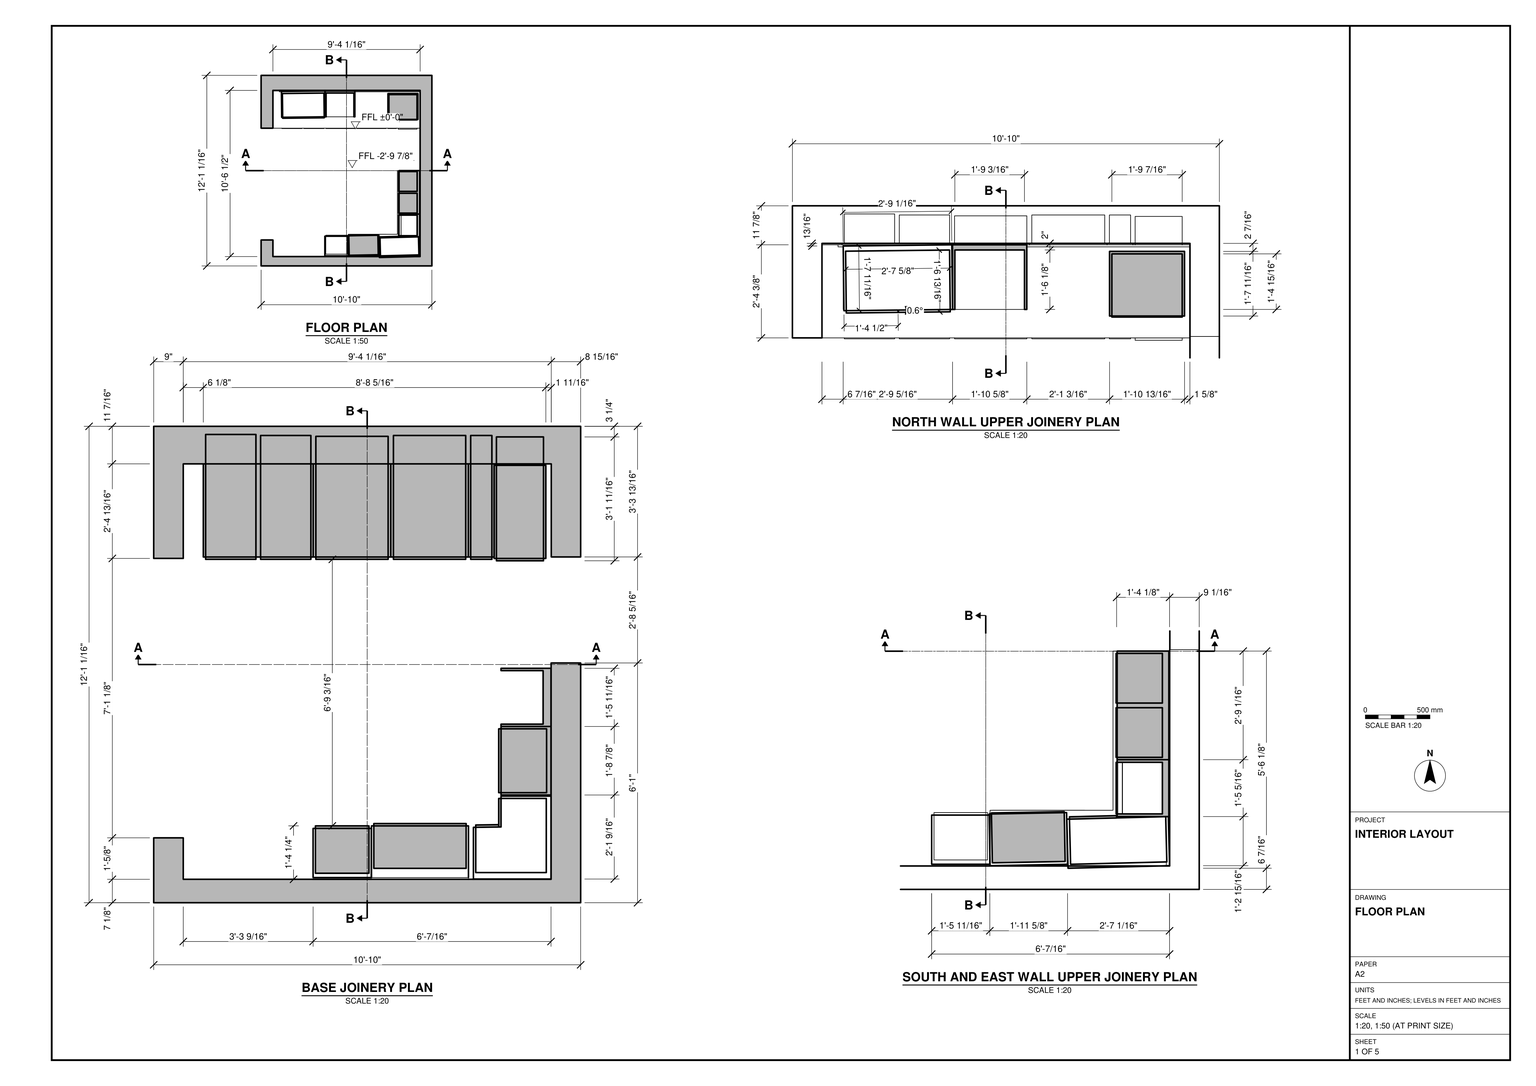
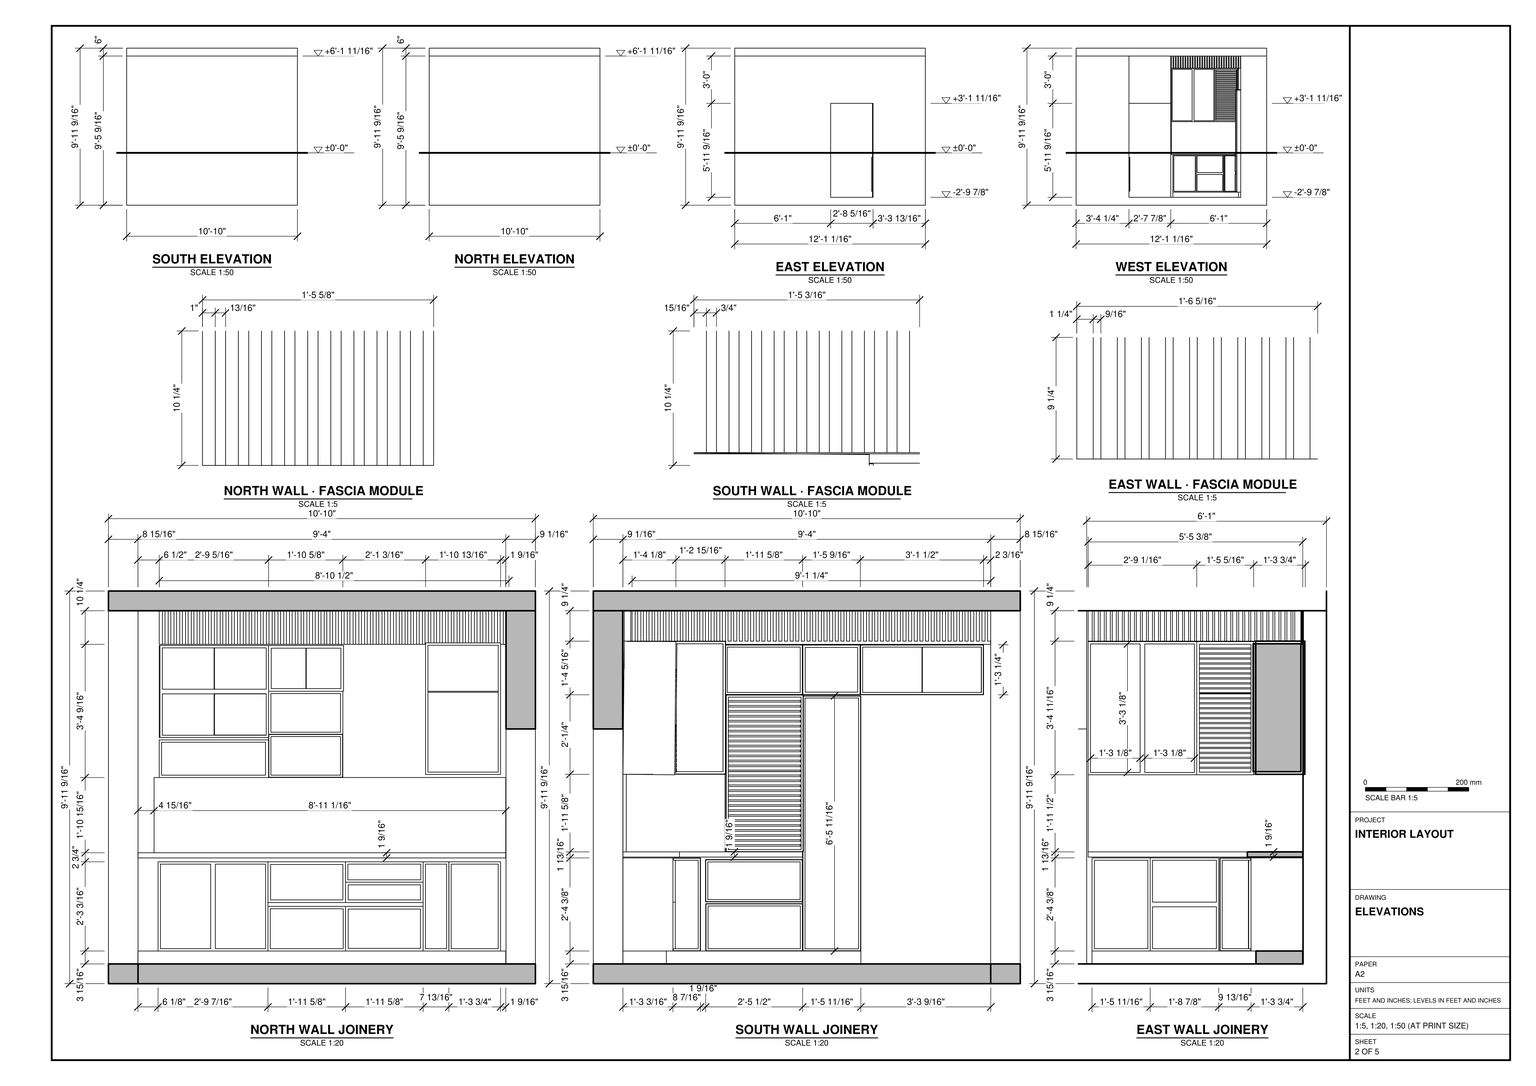
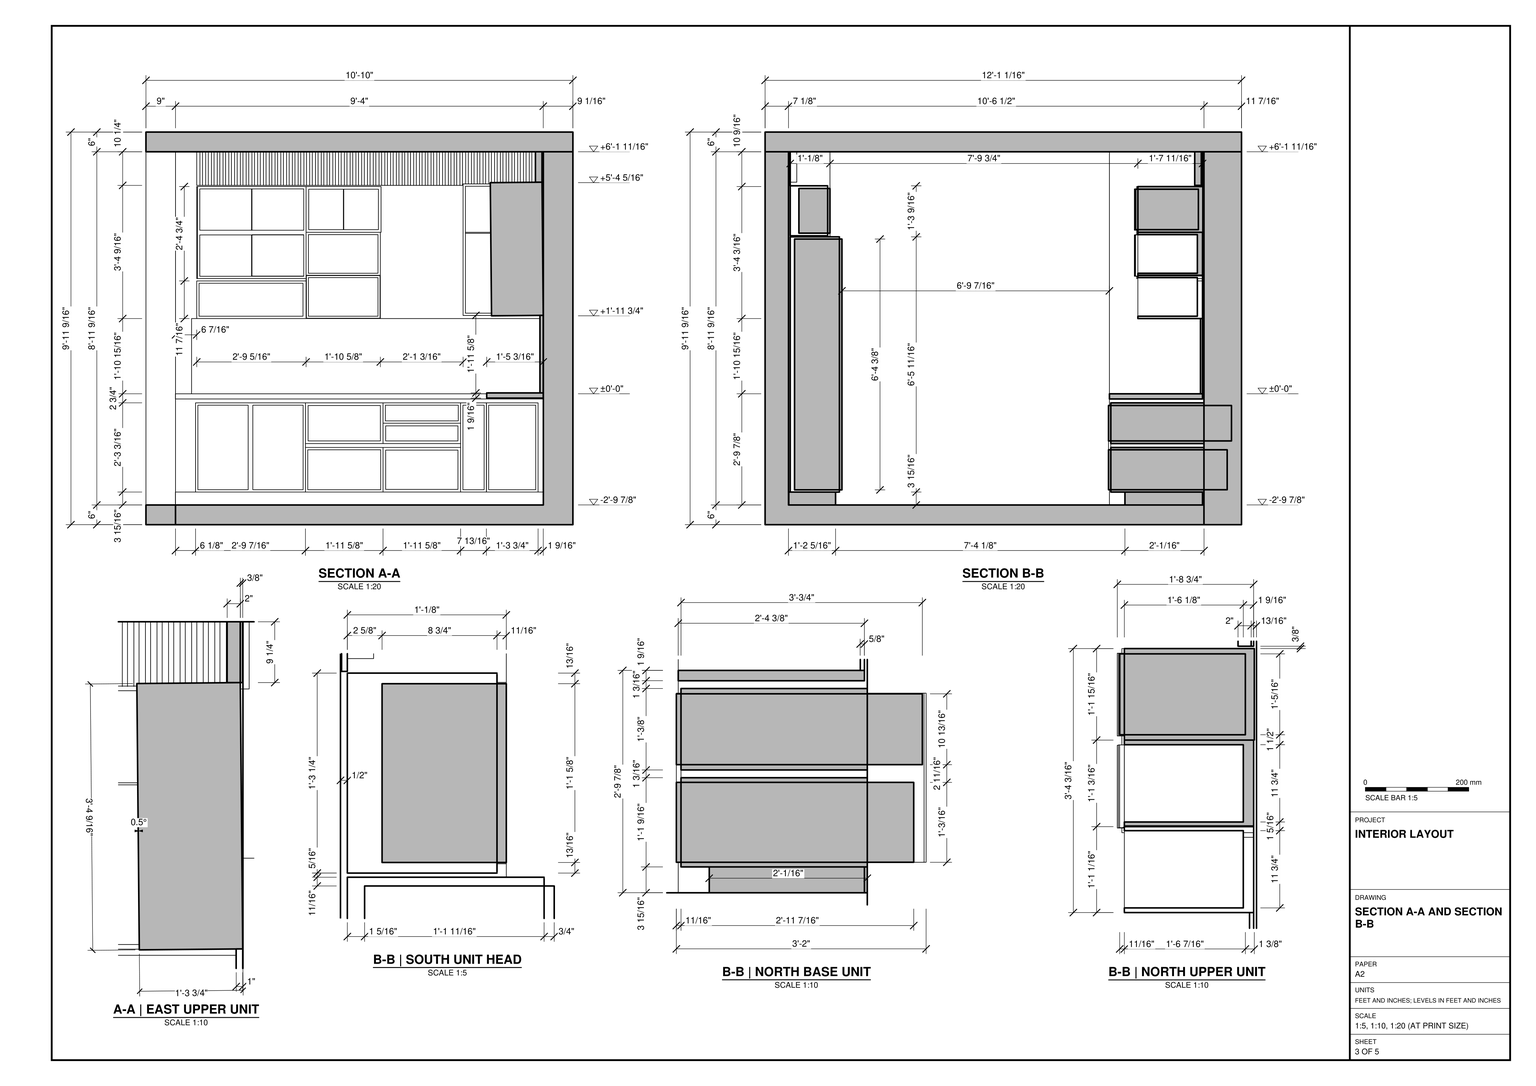
Build the room and its fitted cabinetry in SketchUp from task_files/diagram_01.pdf. Work in feet and inches. Set the outside dimensions to 10'-10" east to west, 12'-1 1/16" north to south and 9'-11 9/16" high. Use the single-storey datum ±0'-0" at the north worktop; the finished floor is at -2'-9 7/8" in the sections.

Model the floor slab, overhead slab and walls with their thicknesses as drawn. Leave the wide opening between the west wall returns and form the narrower opening in the east wall. Use the base and upper joinery plans separately: the cabinet footprints change with height. On the north wall, model the recessed plinth, base cabinets, drawer fronts and continuous worktop. Above it, build the divided upper cabinets and leave the gap before the right-hand unit. Fit the other cabinet run around the south-east corner, matching the tall unit, overhead cabinets and horizontally slatted fronts to the elevations. Distinguish those fronts from the vertically ribbed fascia above the cabinetry.

Keep the walls, slabs and each joinery piece in separate groups or components, and use components for repeated parts. Any decor or loose items shown may be represented by suitable library components. Save one SketchUp model as output_files/room_shell_and_three_wall_cabinet_fit_out.skp.

# SketchUp Ruby script. Lengths in inches.
U = 1.inch
M = Sketchup.active_model
def pt(a) = Geom::Point3d.new(a.map { |v| v * U })
def face(e, loops, mat)
  f = e.add_face(loops[0].map { |a| pt(a) })
  loops[1..].each { |l| e.add_face(l.map { |a| pt(a) }).erase! }
  f.material = f.back_material = mat if mat
  f
end
# faces: each face lists its corners as indices into pts; further lists are holes
def faces(e, pts, list, mat = nil) = list.each { |f| face(e, (f[0].is_a?(Array) ? f : [f]).map { |l| l.map { |i| pts[i] } }, mat) }
# xy, xz, yz: faces in a plane at the given z, y or x. An outline is a flat list of corners, or four numbers for a rectangle; further outlines are holes
def ring(l) = l.size == 4 ? [[l[0], l[1]], [l[2], l[1]], [l[2], l[3]], [l[0], l[3]]] : l.each_slice(2).to_a
def flat(e, list, mat, &to3) = list.each { |f| face(e, (f[0].is_a?(Array) ? f : [f]).map { |l| ring(l).map { |u, v| to3.(u, v) } }, mat) }
def xy(e, z, list, mat = nil) = flat(e, list, mat) { |x, y| [x, y, z] }
def xz(e, y, list, mat = nil) = flat(e, list, mat) { |x, z| [x, y, z] }
def yz(e, x, list, mat = nil) = flat(e, list, mat) { |y, z| [x, y, z] }
def lines(e, pts, list) = list.each { |a, b| e.add_line(pt(pts[a]), pt(pts[b])) }
# prism: a flat outline (further loops are holes) pulled along v
def prism(e, loops, v, mat = nil)
  f = face(e, loops, mat); d = Geom::Vector3d.new(v.map { |x| x * U })
  f.pushpull(f.normal.samedirection?(d) ? d.length : -d.length)
end
def box(e, o, s, mat = nil) = prism(e, [[o, [o[0] + s[0], o[1], o[2]], [o[0] + s[0], o[1] + s[1], o[2]], [o[0], o[1] + s[1], o[2]]]], [0, 0, s[2]], mat)
def at(x, y, z, deg = 0) = Geom::Transformation.translation(pt([x, y, z])) * Geom::Transformation.rotation(ORIGIN, Z_AXIS, deg.degrees)
def axes(o, x, y, z) = Geom::Transformation.new([*x, 0, *y, 0, *z, 0, *pt(o).to_a, 1])
def part(name) = M.definitions.add(name)
# library, detail: a bought-in or finely detailed component or shape, given as its bounding box
def library(name, o, s) = part(name).tap { |d| box(d.entities, o, s) }
def detail(e, o, s) = box(e.add_group.entities, o, s)
def put(e, d, t, mat = nil) = e.add_instance(d, t).tap { |i| i.material = mat if mat }
def group(e, t, mat = nil) = e.add_group.tap { |g| g.transformation = t; g.material = mat if mat }.entities
root = M.entities
M.materials.add("Teddy_Bracelet").color = [145, 141, 147]
M.materials.add("Teddy_DressDepth").color = [117, 194, 193]
M.materials.add("Teddy_Skin ").color = [196, 161, 133]
M.materials.add("[Color B03]").color = [201, 127, 109]
M.materials.add("[Color H06]").color = [158, 204, 204]
M.materials.add("[Color M00]").color = [255, 255, 255]
M.materials.add("[Color M04]").color = [142, 142, 142]
M.materials.add("[Metal Steel Textured]").color = [106, 110, 123]
M.materials.add("[Translucent Glass Sky Reflection]").color = [126, 138, 183]
M.materials["[Translucent Glass Sky Reflection]"].alpha = 0.52
M.materials.add("[Wood Veneer 01]").color = [120, 70, 37]
M.materials.add("[Wood Veneer 02]").color = [190, 128, 91]
c1 = part("Group\#46")
box(c1.entities,[0,-2,0],[0.97,2,10.24])
c2 = part("Group\#68")
box(c2.entities,[-2,0,0],[2,1.25,9.26])
c3 = part("Group\#58")
prism(c3.entities,[[[1.5,0,-0.15],[1.5,15.12,-0.15],[13.78,15.12,-0.04],[13.78,0,-0.04]]],[0,0,0.52])
c4 = part("Group\#62")
prism(c4.entities,[[[1.5,0,-0.34],[1.5,15.71,-0.34],[13.78,15.71,-0.23],[13.78,0,-0.23]]],[-0.01,0,0.71])
c5 = part("Group\#63")
g1 = group(c5.entities,at(0,0,0))
prism(g1,[[[0.01,15.71,0],[0.01,0,0],[-0.15,0,0],[-0.15,15.71,0]]],[-0.01,0,1.12])
c6 = part("Group\#75")
box(c6.entities,[0,0,0],[0.95,2,9.26])
c7 = part("Group\#84")
prism(c7.entities,[[[22.17,0.41,0],[0,0,0],[-0.01,0.31,0],[22.17,0.73,0]]],[0,0,1.04])
xy(root,4.08,[[8.97,109.58,15.07,133.2]])
p = [[66.32,7.22,82.11],[66.32,7.65,97.47],[89.91,7.65,97.47],[89.91,7.22,82.11]]
faces(root,p,[[0,1,2,3]])
g2 = group(root,at(8.97,95.84,0.14))
box(g2,[0,13.74,0],[112.01,23.62,3.9375])
g3 = group(root,at(103.65,109.58,4.08))
xy(g3,0,[[0,-4.74,15.75,23.62]])
xy(g3,0.71,[[0.71,-4.74,15.04,32.27]])
xy(g3,26.46,[[0.71,-4.74,15.04,32.27]])
xy(g3,27.17,[[0,-4.74,15.75,23.62]])
xz(g3,-4.74,[[[0,0,15.75,27.17],[0.71,0.71,15.04,26.46]]])
xz(g3,23.62,[[0,0,15.75,27.17]])
xz(g3,32.27,[[0.71,0.71,15.04,26.46]])
yz(g3,0,[[-4.74,0,23.62,27.17]])
yz(g3,0.71,[[-4.74,0.71,32.27,26.46]])
yz(g3,15.04,[[-4.74,0.71,32.27,26.46]])
yz(g3,15.75,[[-4.74,0,23.62,27.17]])
g4 = group(g3,at(0.71,-4.74,0.71),"[Color B03]")
box(g4,[0,-0.71,0],[14.33,0.71,25.75],"[Color H06]")
g5 = group(root,at(8.97,104.84,30.07))
box(g5,[0,0.02,2.36],[112.01,28.34,1.58])
g6 = group(root,at(0,2.76,-5.86))
g7 = group(g6,at(0,0,6))
g8 = group(g7,at(48.57,104.52,3.9375))
xy(g8,0,[[0,-2,23.62,26.36]])
xy(g8,0.71,[[0.71,-2,22.91,33.43]])
xy(g8,12.875,[[0.71,-2,22.91,33.43]])
xy(g8,13.58,[[0,-2,23.62,26.36]])
xz(g8,-2,[[[0,0,23.62,13.58],[0.71,0.71,22.91,12.875]]])
xz(g8,26.36,[[0,0,23.62,13.58]])
xz(g8,33.43,[[0.71,0.71,22.91,12.875]])
yz(g8,0,[[-2,0,26.36,13.58]])
yz(g8,0.71,[[-2,0.71,33.43,12.875]])
yz(g8,22.91,[[-2,0.71,33.43,12.875]])
yz(g8,23.62,[[-2,0,26.36,13.58]])
g9 = group(g8,at(0.71,-2,0.71),"[Color B03]")
box(g9,[0,-0.71,0],[22.2,0.71,12.17],"[Color H06]")
g10 = group(g7,at(72.1875,104.52,3.9375))
xy(g10,0,[[0,-2,23.62,26.36]])
xy(g10,0.81,[[0.81,-2,22.81,35.01]])
xy(g10,12.78,[[0.81,-2,22.81,35.01]])
xy(g10,13.58,[[0,-2,23.62,26.36]])
xz(g10,-2,[[[0,0,23.62,13.58],[0.81,0.81,22.81,12.78]]])
xz(g10,26.36,[[0,0,23.62,13.58]])
xz(g10,35.01,[[0.81,0.81,22.81,12.78]])
yz(g10,0,[[-2,0,26.36,13.58]])
yz(g10,0.81,[[-2,0.81,35.01,12.78]])
yz(g10,22.81,[[-2,0.81,35.01,12.78]])
yz(g10,23.62,[[-2,0,26.36,13.58]])
g11 = group(g10,at(0.81,-2,0.81),"[Color B03]")
box(g11,[0,-0.71,0],[22.01,0.71,11.97],"[Color H06]")
g12 = group(g7,at(48.57,104.52,18.7))
xy(g12,0,[[0,-2,23.62,26.36]])
xy(g12,0.81,[[0.81,-2,22.81,34.75]])
xy(g12,11.59,[[0.81,-2,22.81,34.75]])
xy(g12,12.4,[[0,-2,23.62,26.36]])
xz(g12,-2,[[[0,0,23.62,12.4],[0.81,0.81,22.81,11.59]]])
xz(g12,26.36,[[0,0,23.62,12.4]])
xz(g12,34.75,[[0.81,0.81,22.81,11.59]])
yz(g12,0,[[-2,0,26.36,12.4]])
yz(g12,0.81,[[-2,0.81,34.75,11.59]])
yz(g12,22.81,[[-2,0.81,34.75,11.59]])
yz(g12,23.62,[[-2,0,26.36,12.4]])
g13 = group(g12,at(0.81,-2,0.81),"[Color B03]")
box(g13,[0,-0.71,0],[22.01,0.71,10.79],"[Color H06]")
g14 = group(g7,at(72.1875,104.52,18.7))
xy(g14,0,[[0,-2,23.62,26.36]])
xy(g14,0.81,[[0.81,-2,22.81,35.01]])
xy(g14,5.39,[[0.81,-2,22.81,35.01]])
xy(g14,6.2,[[0,-2,23.62,26.36]])
xz(g14,-2,[[[0,0,23.62,6.2],[0.81,0.81,22.81,5.39]]])
xz(g14,26.36,[[0,0,23.62,6.2]])
xz(g14,35.01,[[0.81,0.81,22.81,5.39]])
yz(g14,0,[[-2,0,26.36,6.2]])
yz(g14,0.81,[[-2,0.81,35.01,5.39]])
yz(g14,22.81,[[-2,0.81,35.01,5.39]])
yz(g14,23.62,[[-2,0,26.36,6.2]])
g15 = group(g14,at(0.81,-2,0.81),"[Color B03]")
box(g15,[0,-0.71,0],[22.01,0.71,4.59],"[Color H06]")
g16 = group(g7,at(95.8125,104.52,3.9375))
xy(g16,0,[[0,-2,7.875,26.36]])
xy(g16,0.71,[[0.71,-2,7.17,35.01]])
xy(g16,26.46,[[0.71,-2,7.17,35.01]])
xy(g16,27.17,[[0,-2,7.875,26.36]])
xz(g16,-2,[[[0,0,7.875,27.17],[0.71,0.71,7.17,26.46]]])
xz(g16,26.36,[[0,0,7.875,27.17]])
xz(g16,35.01,[[0.71,0.71,7.17,26.46]])
yz(g16,0,[[-2,0,26.36,27.17]])
yz(g16,0.71,[[-2,0.71,35.01,26.46]])
yz(g16,7.17,[[-2,0.71,35.01,26.46]])
yz(g16,7.875,[[-2,0,26.36,27.17]])
g17 = group(g16,at(0.71,-2,0.71),"[Color B03]")
box(g17,[0,-0.71,0],[6.46,0.71,25.75],"[Color H06]")
g18 = group(g7,at(72.1875,104.52,24.9))
xy(g18,0,[[0,-2,23.62,26.36]])
xy(g18,0.71,[[0.71,-2,22.91,35.01]])
xy(g18,5.49,[[0.71,-2,22.91,35.01]])
xy(g18,6.2,[[0,-2,23.62,26.36]])
xz(g18,-2,[[[0,0,23.62,6.2],[0.71,0.71,22.91,5.49]]])
xz(g18,26.36,[[0,0,23.62,6.2]])
xz(g18,35.01,[[0.71,0.71,22.91,5.49]])
yz(g18,0,[[-2,0,26.36,6.2]])
yz(g18,0.71,[[-2,0.71,35.01,5.49]])
yz(g18,22.91,[[-2,0.71,35.01,5.49]])
yz(g18,23.62,[[-2,0,26.36,6.2]])
g19 = group(g18,at(0.71,-2,0.71),"[Color H06]")
box(g19,[0,-0.71,0],[22.2,0.71,4.78])
g20 = group(g7,at(15.1,104.52,3.9375))
xy(g20,0,[[0,-2,33.46,26.36]])
xy(g20,0.71,[[0.71,-2,16.02,35.32],[17.44,-2,32.76,35.01]])
xy(g20,26.46,[[0.71,-2,16.02,35.32],[17.44,-2,32.76,35.01]])
xy(g20,27.17,[[0,-2,33.46,26.36]])
xz(g20,-2,[[[0,0,33.46,27.17],[0.71,0.71,16.02,26.46],[17.44,0.71,32.76,26.46]]])
xz(g20,26.36,[[0,0,33.46,27.17]])
xz(g20,35.01,[[17.44,0.71,32.76,26.46]])
xz(g20,35.32,[[0.71,0.71,16.02,26.46]])
yz(g20,0,[[-2,0,26.36,27.17]])
yz(g20,0.71,[[-2,0.71,35.32,26.46]])
yz(g20,16.02,[[-2,0.71,35.32,26.46]])
yz(g20,17.44,[[-2,0.71,35.01,26.46]])
yz(g20,32.76,[[-2,0.71,35.01,26.46]])
yz(g20,33.46,[[-2,0,26.36,27.17]])
g21 = group(g20,at(0.71,-2,0.71),"[Color B03]")
box(g21,[0,-0.71,0],[15.31,0.71,25.75],"[Color H06]")
g22 = group(g20,at(17.44,-2,0.71))
box(g22,[0,-0.71,0],[15.31,0.71,25.75],"[Color H06]")
g23 = group(g7,at(0,0,-6))
xy(g23,0,[[0,-2.76,0,142.32,130.01,142.32,130.01,130.88,121.01,130.88,121.01,-2.76],[121.01,-2.76,130.01,130.88]])
xy(g23,6,[[9,4.375,121.01,4.375,121.01,70.25,130.01,70.25,130.01,102.54,121.06,102.54,121.06,130.88,9,130.88],[0,17,9,102.1]])
xy(g23,77.56,[[121.06,70.25,130.01,102.54]])
xy(g23,113.56,[[0,-2.76,130.01,-2.76,130.01,142.32,0,142.32,0,102.1,9,102.1,9,130.88,121.06,130.88,121.06,70.25,121.01,70.25,121.01,4.375,9,4.375,9,17,0,17],[0,17,9,102.1]])
xz(g23,-2.76,[[0,0,130.01,113.56]])
xz(g23,4.375,[[9,6,121.01,113.56]],"Teddy_Bracelet")
xz(g23,17,[[0,6,9,113.56]])
xz(g23,70.25,[[121.01,6,121.01,113.56,121.06,113.56,121.06,77.56,130.01,77.56,130.01,6]])
xz(g23,102.1,[[0,6,9,113.56]])
xz(g23,102.54,[[121.06,6,130.01,77.56]])
xz(g23,130.88,[[9,0,121.01,6]])
xz(g23,130.88,[[9,6,121.06,113.56]],"Teddy_Bracelet")
xz(g23,142.32,[[0,0,130.01,113.56]])
yz(g23,0,[[-2.76,0,-2.76,113.56,17,113.56,17,6,102.1,6,102.1,113.56,142.32,113.56,142.32,0]])
yz(g23,9,[[9,0,130.88,6]])
yz(g23,9,[[4.375,6,17,113.56],[102.1,6,130.88,113.56]],"Teddy_Bracelet")
yz(g23,121.01,[[4.375,6,70.25,113.56]])
yz(g23,121.06,[[102.54,6,102.54,77.56,70.25,77.56,70.25,113.56,130.88,113.56,130.88,6]],"Teddy_Bracelet")
yz(g23,130.01,[[[-2.76,0,142.32,113.56],[70.25,6,102.54,77.56]]])
p = [[130.01,130.88,6],[121.06,130.88,6],[0,4.9,6],[9,4.9,6]]
lines(g23,p,[[0,1],[2,3]])
g24 = group(root,at(13.89,133.2,34))
box(g24,[0,-0.625,0],[107.09,0.625,22.91])
g25 = group(root,at(15.46,133.2,97.47),"[Wood Veneer 02]")
box(g25,[0,-0.375,0],[106.49,0.375,10.24])
g26 = group(root,at(15.46,133.2,56.92))
xy(g26,0,[[0,-19.69,33.29,0]])
xy(g26,0.71,[[0.71,-19.69,32.36,-1.57]])
xy(g26,10.75,[[0.71,-19.69,32.36,-1.57]])
xy(g26,11.46,[[0,-19.69,33.29,0]])
xz(g26,-19.69,[[[0,0,33.29,11.46],[0.71,0.71,32.36,10.75]]])
xz(g26,-1.57,[[0.71,0.71,32.36,10.75]])
xz(g26,0,[[0,0,33.29,11.46]])
yz(g26,0,[[-19.69,0,0,11.46]])
yz(g26,0.71,[[-19.69,0.71,-1.57,10.75]])
yz(g26,32.36,[[-19.69,0.71,-1.57,10.75]])
yz(g26,33.29,[[-19.69,0,0,11.46]])
g27 = group(root,at(15.46,132.83,68.73),"[Color M00]")
xy(g27,0.35,[[0.22,-19.68,0,0,33.07,0.375,33.29,-19.31]])
xy(g27,1.0625,[[0.93,-19.68,32.59,-19.32,32.38,-1.21,0.73,-1.57]])
xy(g27,13.66,[[0.93,-19.68,0.73,-1.57,32.38,-1.21,32.59,-19.32]])
xy(g27,15.08,[[0.93,-19.68,32.59,-19.32,32.38,-1.21,0.73,-1.57]])
xy(g27,27.68,[[0.93,-19.68,0.73,-1.57,32.38,-1.21,32.59,-19.32]])
xy(g27,28.39,[[0.22,-19.68,33.29,-19.31,33.07,0.375,0,0]])
p = [[0,0,28.39],[0,0,0.35],[0.22,-19.68,0.35],[0.22,-19.68,28.39],[33.29,-19.31,28.39],[33.29,-19.31,0.35],
  [0.93,-19.68,15.08],[0.93,-19.68,27.68],[32.59,-19.32,27.68],[32.59,-19.32,15.08],[0.93,-19.68,13.66],[32.59,-19.32,13.66],
  [32.59,-19.32,1.0625],[0.93,-19.68,1.0625],[33.07,0.375,0.35],[33.07,0.375,28.39],[0.73,-1.57,1.0625],[0.73,-1.57,13.66],
  [32.38,-1.21,13.66],[32.38,-1.21,1.0625],[0.73,-1.57,15.08],[0.73,-1.57,27.68],[32.38,-1.21,27.68],[32.38,-1.21,15.08]]
faces(g27,p,[[0,1,2,3],[[4,3,2,5],[6,7,8,9],[10,11,12,13]],[14,15,4,5],[15,14,1,0],[10,13,16,17],[12,11,18,19],[18,17,16,19],[7,6,20,21],
  [9,8,22,23],[21,20,23,22]])
g28 = group(g27,at(0.93,-19.68,15.08))
prism(g28,[[[0,0,0],[15.76,0.18,0],[15.77,-0.53,0],[0.01,-0.71,0]]],[0,0,12.6],"[Color H06]")
prism(g28,[[[0,0,-14.02],[15.76,0.18,-14.02],[15.77,-0.53,-14.02],[0.01,-0.71,-14.02]]],[0,0,12.6],"[Color H06]")
g29 = group(g27,at(16.82,-19.5,15.08))
prism(g29,[[[0,0,0],[15.76,0.18,0],[15.77,-0.53,0],[0.01,-0.71,0]]],[0,0,12.6],"[Color H06]")
prism(g29,[[[0,0,-13.96],[15.76,0.18,-13.96],[15.77,-0.53,-13.96],[0.01,-0.71,-13.96]]],[0,0,12.6],"[Color H06]")
g30 = group(root,at(48.76,133.2,56.92))
xy(g30,0,[[0,-19.68,22.61,0]])
xy(g30,0.71,[[0.71,-19.68,21.9,-1.57]])
xy(g30,12.47,[[0.71,-19.68,21.9,-1.57]])
xy(g30,13.18,[[0,-19.68,22.61,0]])
xz(g30,-19.68,[[[0.1,0.1,22.51,13.08],[0.71,0.71,21.9,12.47]]])
xz(g30,-1.57,[[0.71,0.71,21.9,12.47]])
xz(g30,0,[[0,0,22.61,13.18]])
yz(g30,0.71,[[-19.68,0.71,-1.57,12.47]])
yz(g30,21.9,[[-19.68,0.71,-1.57,12.47]])
yz(g30,22.61,[[-19.68,0,0,13.18]])
g31 = group(root,at(48.76,133.2,70))
xy(g31,0,[[0,-19.68,22.61,0]])
xy(g31,0.71,[[0.71,-19.68,21.9,-1.57]])
xy(g31,12.47,[[0.71,-19.68,21.9,-1.57]])
xy(g31,13.18,[[0,-19.68,22.61,0]])
xz(g31,-19.68,[[[0,0,22.61,13.18],[0.71,0.71,21.9,12.47]]])
xz(g31,-1.57,[[0.71,0.71,21.9,12.47]])
xz(g31,0,[[0,0,22.61,13.18]])
yz(g31,0,[[-19.68,0,0,13.18]])
yz(g31,0.71,[[-19.68,0.71,-1.57,12.47]])
yz(g31,21.9,[[-19.68,0.71,-1.57,12.47]])
yz(g31,22.61,[[-19.68,0,0,13.18]])
g32 = group(root,at(48.76,133.3,83.18),"[Color M00]")
xy(g32,0,[[0,-19.79,22.83,0]])
xy(g32,0.81,[[0.81,-19.79,22.03,-1.36]])
xy(g32,13.125,[[0.81,-19.79,22.03,-1.36]])
xy(g32,13.93,[[0,-19.79,22.83,0]])
xz(g32,-19.79,[[[0,0,22.83,13.93],[0.81,0.81,22.03,13.125]]])
xz(g32,-1.36,[[0.81,0.81,22.03,13.125]])
xz(g32,0,[[0,0,22.83,13.93]])
yz(g32,0,[[-19.79,0,0,13.93]])
yz(g32,0.81,[[-19.79,0.81,-1.36,13.125]])
yz(g32,22.03,[[-19.79,0.81,-1.36,13.125]])
yz(g32,22.83,[[-19.79,0,0,13.93]])
g33 = group(root,at(49.5625,113.52,83.99))
box(g33,[0,-0.71,0],[10.55,0.71,12.32],"[Color H06]")
g34 = group(root,at(60.24,113.52,83.99))
box(g34,[0,-0.71,0],[10.55,0.71,12.32],"[Color H06]")
g35 = group(root,at(96.57,131.2,57.85),"[Color M00]")
xy(g35,0,[[0,-19.69,22.83,0]])
xy(g35,0.71,[[0.71,-19.69,22.125,-0.76]])
xy(g35,39.35,[[0.71,-19.69,22.125,-0.76]])
xy(g35,40.06,[[0,-19.69,22.83,0]])
xz(g35,-19.69,[[[0,0,22.83,40.06],[0.71,0.71,22.125,39.35]]],"[Metal Steel Textured]")
xz(g35,-0.76,[[0.71,0.71,22.125,39.35]])
xz(g35,0,[[0,0,22.83,40.06]])
yz(g35,0,[[-19.69,0,0,40.06]])
yz(g35,0.71,[[-19.69,0.71,-0.76,39.35]])
yz(g35,22.125,[[-19.69,0.71,-0.76,39.35]])
yz(g35,22.83,[[-19.69,0,0,40.06]])
g36 = group(g35,at(0.71,-19.69,12.52))
box(g36,[0,2,-0.35],[21.42,16.92,0.7])
g37 = group(g35,at(0.71,-19.69,24.33))
box(g37,[0,2,-0.35],[21.42,16.92,0.7])
g38 = group(root,at(97.27,111.52,83.18))
box(g38,[0,-0.31,0],[21.42,0.31,14.02],"[Translucent Glass Sky Reflection]")
g39 = group(root,at(97.27,111.52,58.5625))
box(g39,[0,-0.31,0],[21.42,0.31,24.31],"[Translucent Glass Sky Reflection]")
put(root,c1,at(15.46,132.83,97.47),"[Wood Veneer 02]")
put(root,c1,at(17.22,132.83,97.47),"[Wood Veneer 02]")
put(root,c1,at(18.98,132.83,97.47),"[Wood Veneer 02]")
put(root,c1,at(20.74,132.83,97.47),"[Wood Veneer 02]")
put(root,c1,at(22.5,132.83,97.47),"[Wood Veneer 02]")
put(root,c1,at(24.26,132.83,97.47),"[Wood Veneer 02]")
put(root,c1,at(26.02,132.83,97.47),"[Wood Veneer 02]")
put(root,c1,at(27.78,132.83,97.47),"[Wood Veneer 02]")
put(root,c1,at(29.54,132.83,97.47),"[Wood Veneer 02]")
put(root,c1,at(31.3,132.83,97.47),"[Wood Veneer 02]")
put(root,c1,at(33.06,132.83,97.47),"[Wood Veneer 02]")
put(root,c1,at(34.82,132.83,97.47),"[Wood Veneer 02]")
put(root,c1,at(36.58,132.83,97.47),"[Wood Veneer 02]")
put(root,c1,at(38.33,132.83,97.47),"[Wood Veneer 02]")
put(root,c1,at(40.09,132.83,97.47),"[Wood Veneer 02]")
put(root,c1,at(41.85,132.83,97.47),"[Wood Veneer 02]")
put(root,c1,at(43.61,132.83,97.47),"[Wood Veneer 02]")
put(root,c1,at(45.37,132.83,97.47),"[Wood Veneer 02]")
put(root,c1,at(47.13,132.83,97.47),"[Wood Veneer 02]")
put(root,c1,at(48.89,132.83,97.47),"[Wood Veneer 02]")
put(root,c1,at(50.65,132.83,97.47),"[Wood Veneer 02]")
put(root,c1,at(52.41,132.83,97.47),"[Wood Veneer 02]")
put(root,c1,at(54.17,132.83,97.47),"[Wood Veneer 02]")
put(root,c1,at(55.93,132.83,97.47),"[Wood Veneer 02]")
put(root,c1,at(57.6875,132.83,97.47),"[Wood Veneer 02]")
put(root,c1,at(59.45,132.83,97.47),"[Wood Veneer 02]")
put(root,c1,at(61.21,132.83,97.47),"[Wood Veneer 02]")
put(root,c1,at(62.97,132.83,97.47),"[Wood Veneer 02]")
put(root,c1,at(64.73,132.83,97.47),"[Wood Veneer 02]")
put(root,c1,at(66.48,132.83,97.47),"[Wood Veneer 02]")
put(root,c1,at(68.24,132.83,97.47),"[Wood Veneer 02]")
put(root,c1,at(70,132.83,97.47),"[Wood Veneer 02]")
put(root,c1,at(71.76,132.83,97.47),"[Wood Veneer 02]")
put(root,c1,at(73.52,132.83,97.47),"[Wood Veneer 02]")
put(root,c1,at(75.28,132.83,97.47),"[Wood Veneer 02]")
put(root,c1,at(77.04,132.83,97.47),"[Wood Veneer 02]")
put(root,c1,at(78.8,132.83,97.47),"[Wood Veneer 02]")
put(root,c1,at(80.56,132.83,97.47),"[Wood Veneer 02]")
put(root,c1,at(82.32,132.83,97.47),"[Wood Veneer 02]")
put(root,c1,at(84.08,132.83,97.47),"[Wood Veneer 02]")
put(root,c1,at(85.84,132.83,97.47),"[Wood Veneer 02]")
put(root,c1,at(87.6,132.83,97.47),"[Wood Veneer 02]")
put(root,c1,at(89.36,132.83,97.47),"[Wood Veneer 02]")
put(root,c1,at(91.12,132.83,97.47),"[Wood Veneer 02]")
put(root,c1,at(92.875,132.83,97.47),"[Wood Veneer 02]")
put(root,c1,at(94.63,132.83,97.47),"[Wood Veneer 02]")
put(root,c1,at(96.39,132.83,97.47),"[Wood Veneer 02]")
put(root,c1,at(98.15,132.83,97.47),"[Wood Veneer 02]")
put(root,c1,at(99.91,132.83,97.47),"[Wood Veneer 02]")
put(root,c1,at(101.67,132.83,97.47),"[Wood Veneer 02]")
put(root,c1,at(103.43,132.83,97.47),"[Wood Veneer 02]")
put(root,c1,at(105.19,132.83,97.47),"[Wood Veneer 02]")
put(root,c1,at(106.95,132.83,97.47),"[Wood Veneer 02]")
put(root,c1,at(108.71,132.83,97.47),"[Wood Veneer 02]")
put(root,c1,at(110.47,132.83,97.47),"[Wood Veneer 02]")
put(root,c1,at(112.23,132.83,97.47),"[Wood Veneer 02]")
put(root,c1,at(113.99,132.83,97.47),"[Wood Veneer 02]")
put(root,c1,at(115.75,132.83,97.47),"[Wood Veneer 02]")
put(root,c1,at(117.51,132.83,97.47),"[Wood Veneer 02]")
put(root,c1,at(119.27,132.83,97.47),"[Wood Veneer 02]")
g40 = group(root,at(105.76,7.22,0.14))
prism(g40,[[[15.21,0,0],[-57.23,0,0],[-57.23,14.25,0],[2,14.25,0],[2,64.17,0],[15.21,64.17,0]]],[0,0,3.9375])
g41 = group(root,at(105.76,53.67,4.08))
xy(g41,0,[[0,0,15.21,17.72]])
xy(g41,0.71,[[0,0.71,12.8125,17.01]])
xy(g41,27.64,[[0,0.71,12.8125,17.01]])
xy(g41,28.35,[[0,0,15.21,17.72]])
xz(g41,0,[[0,0,15.21,28.35]])
xz(g41,0.71,[[0,0.71,12.8125,27.64]])
xz(g41,17.01,[[0,0.71,12.8125,27.64]])
xz(g41,17.72,[[0,0,15.21,28.35]])
yz(g41,0,[[[0,0,17.72,28.35],[0.71,0.71,17.01,27.64]]])
yz(g41,12.8125,[[0.71,0.71,17.01,27.64]])
yz(g41,15.21,[[0,0,17.72,28.35]])
g42 = group(root,at(105.76,32.81,4.08))
xy(g42,0,[[0,0,15.21,20.87]])
xy(g42,0.71,[[0,0.71,9.4375,20.16]])
xy(g42,13.46,[[0,0.71,9.4375,20.16]])
xy(g42,14.88,[[0,0.71,13.875,20.16]])
xy(g42,27.64,[[0,0.71,13.875,20.16]])
xy(g42,28.35,[[0,0,15.21,20.87]])
xz(g42,0,[[0,0,15.21,28.35]])
xz(g42,0.71,[[0,0.71,9.4375,13.46],[0,14.88,13.875,27.64]])
xz(g42,20.16,[[0,0.71,9.4375,13.46],[0,14.88,13.875,27.64]])
xz(g42,20.87,[[0,0,15.21,28.35]])
yz(g42,0,[[[0,0,20.87,28.35],[0.71,14.88,20.16,27.64],[0.71,0.71,20.16,13.46]]])
yz(g42,9.4375,[[0.71,0.71,20.16,13.46]])
yz(g42,13.875,[[0.71,14.88,20.16,27.64]])
yz(g42,15.21,[[0,0,20.87,28.35]])
g43 = group(g42,at(0,0.71,14.88))
box(g43,[-0.71,0,0],[0.71,19.45,12.76],"[Color H06]")
g44 = group(root,at(107.76,7.22,4.08))
xy(g44,0,[[-10.41,0,-10.41,15.75,-2,15.75,-2,25.25,13.21,25.25,13.21,0]])
xy(g44,0.71,[[-9.7,1.97,11.78,15.75],[-2,15.85,11.78,24.54]])
xy(g44,27.64,[[-9.7,1.97,11.78,15.75],[-2,15.85,11.78,24.54]])
xy(g44,28.35,[[-10.41,0,13.21,0,13.21,25.25,-2,25.25,-2,15.75,-10.41,15.75]])
xz(g44,0,[[-10.41,0,13.21,28.35]])
xz(g44,1.97,[[-9.7,0.71,11.78,27.64]])
xz(g44,15.75,[[-10.31,0.1,-10.31,28.25,-2.1,28.25,-2.1,27.64,-9.7,27.64,-9.7,0.71,-2.1,0.71,-2.1,0.1]])
xz(g44,24.54,[[-2,0.71,11.78,27.64]])
xz(g44,25.25,[[-2,0,13.21,28.35]])
yz(g44,-10.41,[[0,0,15.75,28.35]])
yz(g44,-9.7,[[1.97,0.71,15.75,27.64]])
yz(g44,-2,[[15.85,0.1,15.85,0.71,24.54,0.71,24.54,27.64,15.85,27.64,15.85,28.25,25.15,28.25,25.15,0.1]])
yz(g44,11.78,[[1.97,0.71,15.75,27.64],[15.85,0.71,24.54,27.64]])
yz(g44,13.21,[[0,0,25.25,28.35]])
p = [[-2,15.75,0],[-2,15.75,0.71],[-2,15.75,27.64],[-2,15.75,28.35]]
lines(g44,p,[[0,1],[2,3]])
g45 = group(root,at(105.76,7.22,32.7))
prism(g45,[[[15.21,65.35,0],[15.21,0,0],[-39.44,0,0],[-39.44,16.88,0],[-2,16.88,0],[-2,65.35,0]]],[0,0,1.57])
g46 = group(root,at(120.97,7.22,98.44),"[Wood Veneer 02]")
box(g46,[-0.375,0,0],[0.375,65.35,9.26])
g47 = group(root,at(120.6,71.32,98.44),"[Wood Veneer 02]")
box(g47,[-2,0,0],[2,1.25,9.26])
g48 = group(root,at(120.6,69.49,98.44),"[Wood Veneer 02]")
box(g48,[-2,0,0],[2,1.25,9.26])
put(root,c2,at(120.6,67.65,98.44),"[Wood Veneer 02]")
put(root,c2,at(120.6,65.82,98.44),"[Wood Veneer 02]")
put(root,c2,at(120.6,63.98,98.44),"[Wood Veneer 02]")
put(root,c2,at(120.6,62.15,98.44),"[Wood Veneer 02]")
put(root,c2,at(120.6,60.32,98.44),"[Wood Veneer 02]")
put(root,c2,at(120.6,58.48,98.44),"[Wood Veneer 02]")
put(root,c2,at(120.6,56.65,98.44),"[Wood Veneer 02]")
put(root,c2,at(120.6,54.8125,98.44),"[Wood Veneer 02]")
put(root,c2,at(120.6,52.98,98.44),"[Wood Veneer 02]")
put(root,c2,at(120.6,51.15,98.44),"[Wood Veneer 02]")
put(root,c2,at(120.6,49.3125,98.44),"[Wood Veneer 02]")
put(root,c2,at(120.6,47.48,98.44),"[Wood Veneer 02]")
put(root,c2,at(120.6,45.64,98.44),"[Wood Veneer 02]")
put(root,c2,at(120.6,43.81,98.44),"[Wood Veneer 02]")
put(root,c2,at(120.6,41.98,98.44),"[Wood Veneer 02]")
put(root,c2,at(120.6,40.14,98.44),"[Wood Veneer 02]")
put(root,c2,at(120.6,38.31,98.44),"[Wood Veneer 02]")
put(root,c2,at(120.6,36.47,98.44),"[Wood Veneer 02]")
put(root,c2,at(120.6,34.64,98.44),"[Wood Veneer 02]")
put(root,c2,at(120.6,32.81,98.44),"[Wood Veneer 02]")
put(root,c2,at(120.6,30.97,98.44),"[Wood Veneer 02]")
put(root,c2,at(120.6,29.14,98.44),"[Wood Veneer 02]")
put(root,c2,at(120.6,27.31,98.44),"[Wood Veneer 02]")
put(root,c2,at(120.6,25.47,98.44),"[Wood Veneer 02]")
put(root,c2,at(120.6,23.64,98.44),"[Wood Veneer 02]")
put(root,c2,at(120.6,21.8,98.44),"[Wood Veneer 02]")
put(root,c2,at(120.6,19.97,98.44),"[Wood Veneer 02]")
put(root,c2,at(120.6,18.14,98.44),"[Wood Veneer 02]")
put(root,c2,at(120.6,16.3,98.44),"[Wood Veneer 02]")
put(root,c2,at(120.6,14.47,98.44),"[Wood Veneer 02]")
put(root,c2,at(120.6,12.63,98.44),"[Wood Veneer 02]")
put(root,c2,at(120.6,10.8,98.44),"[Wood Veneer 02]")
put(root,c2,at(120.6,8.97,98.44),"[Wood Veneer 02]")
put(root,c2,at(120.6,7.13,98.44),"[Wood Veneer 01]")
g49 = group(root,at(120.97,7.22,34.27))
box(g49,[-1,0,0],[1,65.35,23.62])
g50 = group(root,at(120.6,39.5,57.89),"[Color M00]")
xz(g50,0,[[-15.37,-0.15,0.375,0,0,40.55,-15.75,40.41]])
xz(g50,0.71,[[-15.38,0.5625,-15.74,39.7,-1.96,39.82,-1.6,0.69]])
xz(g50,15.83,[[-15.38,0.5625,-1.6,0.69,-1.96,39.82,-15.74,39.7]])
xz(g50,17.24,[[-15.38,0.5625,-15.74,39.7,-1.96,39.82,-1.6,0.69]])
xz(g50,32.36,[[-15.38,0.5625,-1.6,0.69,-1.96,39.82,-15.74,39.7]])
xz(g50,33.07,[[-15.37,-0.15,-15.75,40.41,0,40.55,0.375,0]])
p = [[-15.75,33.07,40.41],[-15.37,33.07,-0.15],[-15.37,0,-0.15],[-15.75,0,40.41],[-15.38,32.36,0.5625],[-15.74,32.36,39.7],
  [-15.74,17.24,39.7],[-15.38,17.24,0.5625],[-15.38,15.83,0.5625],[-15.74,15.83,39.7],[-15.74,0.71,39.7],[-15.38,0.71,0.5625],
  [0.375,33.07,0],[0.375,0,0],[0,33.07,40.55],[0,0,40.55],[-1.6,0.71,0.69],[-1.6,15.83,0.69],
  [-1.6,17.24,0.69],[-1.6,32.36,0.69],[-1.96,15.83,39.82],[-1.96,0.71,39.82],[-1.96,32.36,39.82],[-1.96,17.24,39.82]]
faces(g50,p,[[[0,1,2,3],[4,5,6,7],[8,9,10,11]]],"[Metal Steel Textured]")
faces(g50,p,[[12,13,2,1],[12,14,15,13],[8,11,16,17],[4,7,18,19],[20,17,16,21],[22,19,18,23],[10,9,20,21],[6,5,22,23],
  [15,14,0,3]])
put(g50,c3,at(-15.5,17.24,13.67))
put(g50,c3,at(-15.8125,17.24,26.78))
put(g50,c3,at(-15.8125,0.71,26.78))
put(g50,c3,at(-15.5,0.71,13.74))
g51 = group(root,at(104.86,56.74,58.46),"[Color B03]")
prism(g51,[[[0.36,15.12,0],[0.36,0,0],[0.05,0,0],[0.05,15.12,0]]],[-0.36,0,39.13],"[Translucent Glass Sky Reflection]")
g52 = group(root,at(104.86,40.21,58.46),"[Color B03]")
prism(g52,[[[0.36,15.12,0],[0.36,0,0],[0.05,0,0],[0.05,15.12,0]]],[-0.36,0,39.13],"[Translucent Glass Sky Reflection]")
g53 = group(root,at(120.6,22.18,57.89))
xz(g53,0,[[-15.37,-0.15,0.375,0,0,40.55,-15.75,40.41]])
xz(g53,0.81,[[-15.38,0.66,-15.74,39.6,-1.96,39.73,-1.6,0.79]])
xz(g53,16.52,[[-15.38,0.66,-1.6,0.79,-1.96,39.73,-15.74,39.6]])
xz(g53,17.32,[[-15.37,-0.15,-15.75,40.41,0,40.55,0.375,0]])
p = [[-15.75,17.32,40.41],[-15.37,17.32,-0.15],[-15.37,0,-0.15],[-15.75,0,40.41],[-15.74,0.81,39.6],[-15.38,0.81,0.66],
  [-15.38,16.52,0.66],[-15.74,16.52,39.6],[0.375,17.32,0],[0.375,0,0],[0,17.32,40.55],[0,0,40.55],
  [-1.6,0.81,0.79],[-1.6,16.52,0.79],[-1.96,16.52,39.73],[-1.96,0.81,39.73]]
faces(g53,p,[[[0,1,2,3],[4,5,6,7]],[8,9,2,1],[8,10,11,9],[6,5,12,13],[14,13,12,15],[4,7,14,15],[11,10,0,3]])
put(g53,c4,at(-15.45,0.81,8.54))
put(g53,c4,at(-15.53,0.81,16.41))
put(g53,c4,at(-15.6,0.81,24.28))
put(g53,c4,at(-15.67,0.81,32.16))
put(root,c5,at(104.86,22.98,96.37),"[Color M04]")
put(root,c5,at(104.86,22.98,94.86),"[Color M04]")
put(root,c5,at(104.86,22.98,93.34),"[Color M04]")
put(root,c5,at(104.86,22.98,91.83),"[Color M04]")
put(root,c5,at(104.86,22.98,90.32),"[Color M04]")
put(root,c5,at(104.86,22.98,88.81),"[Color M04]")
put(root,c5,at(104.86,22.98,87.29),"[Color M04]")
put(root,c5,at(104.86,22.98,85.78),"[Color M04]")
put(root,c5,at(104.86,22.98,84.27),"[Color M04]")
put(root,c5,at(104.86,22.98,82.76),"[Color M04]")
put(root,c5,at(104.86,22.98,81.24),"[Color M04]")
put(root,c5,at(104.86,22.98,79.73),"[Color M04]")
put(root,c5,at(104.86,22.98,78.22),"[Color M04]")
put(root,c5,at(104.86,22.98,76.71),"[Color M04]")
put(root,c5,at(104.86,22.98,75.19),"[Color M04]")
put(root,c5,at(104.86,22.98,73.68),"[Color M04]")
put(root,c5,at(104.86,22.98,72.17),"[Color M04]")
put(root,c5,at(104.86,22.98,70.66),"[Color M04]")
put(root,c5,at(104.86,22.98,69.14),"[Color M04]")
put(root,c5,at(104.86,22.98,67.63),"[Color M04]")
put(root,c5,at(104.86,22.98,66.12),"[Color M04]")
put(root,c5,at(104.86,22.98,64.61),"[Color M04]")
put(root,c5,at(104.86,22.98,63.09),"[Color M04]")
put(root,c5,at(104.86,22.98,61.58),"[Color M04]")
put(root,c5,at(104.86,22.98,60.07),"[Color M04]")
put(root,c5,at(104.86,22.98,58.56),"[Color M04]")
g54 = group(root,at(120.6,7.22,57.89),"[Color M00]")
xy(g54,0,[[-30.54,-0.77,-30.91,14.1875,0,14.96,0.375,0]])
xy(g54,0.81,[[-29.76,0.43,-0.46,1.17,-0.81,14.94,-15.75,14.57,-30.11,14.21]])
xy(g54,39.74,[[-29.76,0.43,-30.11,14.21,-15.75,14.57,-0.81,14.94,-0.46,1.17]])
xy(g54,40.55,[[-30.54,-0.77,0.375,0,0,14.96,-30.91,14.1875]])
p = [[-30.54,-0.77,0],[-30.54,-0.77,40.55],[-30.91,14.1875,40.55],[-30.91,14.1875,0],[0.375,0,0],[0.375,0,40.55],
  [0,14.96,0],[0,14.96,40.55],[-0.1,14.96,40.45],[-0.1,14.96,0.1],[-30.82,14.1875,0.1],[-30.82,14.1875,40.45],
  [-30.11,14.21,39.74],[-30.11,14.21,0.81],[-15.75,14.57,0.81],[-0.81,14.94,0.81],[-0.81,14.94,39.74],[-15.75,14.57,39.74],
  [-29.76,0.43,39.74],[-29.76,0.43,0.81],[-0.46,1.17,39.74],[-0.46,1.17,0.81]]
faces(g54,p,[[0,1,2,3],[4,5,1,0],[5,4,6,7],[[8,9,10,11],[12,13,14,15,16,17]],[13,12,18,19],[19,18,20,21],[16,15,21,20],[14,17,16,15]])
g55 = group(g54,at(-30.09,14.19,0.81))
prism(g55,[[[14.36,0.36,0],[0,0,0],[-0.02,0.71,0],[14.34,1.07,0]]],[0,0,38.9375],"[Color H06]")
g56 = group(root,at(105.76,23.0625,4.79))
box(g56,[-0.71,0,0],[0.71,8.69,26.93],"Teddy_DressDepth")
g57 = group(g56,at(-7.7,-0.1,0),"[Color H06]")
prism(g57,[[[6.99,0.1,0],[0,0,0],[-0.01,0.71,0],[6.98,0.81,0]]],[0,0,26.93],"[Color H06]")
g58 = group(root,at(66.25,7.65,4.08))
xy(g58,0,[[0,0,29.53,15.75]])
xy(g58,0.71,[[0.71,1.97,28.82,15.75]])
xy(g58,13.71,[[0.71,1.97,28.82,15.75]])
xy(g58,14.42,[[0,0,29.53,15.75]])
xz(g58,0,[[0,0,29.53,14.42]])
xz(g58,1.97,[[0.71,0.71,28.82,13.71]])
xz(g58,15.75,[[[0.1,0.1,29.43,14.32],[0.71,0.71,28.82,13.71]]])
yz(g58,0,[[0,0,15.75,14.42]])
yz(g58,0.71,[[1.97,0.71,15.75,13.71]])
yz(g58,28.82,[[1.97,0.71,15.75,13.71]])
yz(g58,29.53,[[0,0,15.75,14.42]])
g59 = group(g58,at(0.71,15.75,0.71))
box(g59,[0,0,0],[28.11,0.71,13.01],"[Color H06]")
g60 = group(root,at(66.32,7.65,19.04),"[Color M00]")
xy(g60,0.71,[[0.71,2.8125,28.82,15.75]])
xy(g60,12.18,[[0.71,2.8125,28.82,15.75]])
xy(g60,12.89,[[0,0,29.53,15.75]])
xz(g60,2.8125,[[0.71,0.71,28.82,12.18]])
xz(g60,15.75,[[[0.1,0.1,29.43,12.79],[0.71,0.71,28.82,12.18]]])
yz(g60,0,[[0,0,15.75,12.89]])
yz(g60,0.71,[[2.8125,0.71,15.75,12.18]])
yz(g60,28.82,[[2.8125,0.71,15.75,12.18]])
yz(g60,29.53,[[0,0,15.75,12.89]])
p = [[0,15.75,0],[29.53,15.75,0]]
lines(g60,p,[[0,1]])
g61 = group(g60,at(0.71,15.75,0.71))
box(g61,[0,0,0],[28.11,0.71,11.47],"[Color H06]")
g62 = group(root,at(8.97,7.22,97.47),"[Wood Veneer 02]")
box(g62,[0,0,0],[109.23,0.4375,10.24])
put(root,c6,at(117.25,7.65,98.44),"[Wood Veneer 02]")
put(root,c6,at(115.53,7.65,98.44),"[Wood Veneer 02]")
put(root,c6,at(113.8125,7.65,98.44),"[Wood Veneer 02]")
put(root,c6,at(112.1,7.65,98.44),"[Wood Veneer 02]")
put(root,c6,at(110.375,7.65,98.44),"[Wood Veneer 02]")
put(root,c6,at(108.66,7.65,98.44),"[Wood Veneer 02]")
put(root,c6,at(106.94,7.65,98.44),"[Wood Veneer 02]")
put(root,c6,at(105.22,7.65,98.44),"[Wood Veneer 02]")
put(root,c6,at(103.5,7.65,98.44),"[Wood Veneer 02]")
put(root,c6,at(101.79,7.65,98.44),"[Wood Veneer 02]")
put(root,c6,at(100.07,7.65,98.44),"[Wood Veneer 02]")
put(root,c6,at(98.35,7.65,98.44),"[Wood Veneer 02]")
put(root,c6,at(96.63,7.65,98.44),"[Wood Veneer 02]")
put(root,c6,at(94.91,7.65,98.44),"[Wood Veneer 02]")
put(root,c6,at(93.19,7.65,98.44),"[Wood Veneer 02]")
put(root,c6,at(91.48,7.65,98.44),"[Wood Veneer 02]")
put(root,c6,at(89.76,7.65,98.44),"[Wood Veneer 02]")
put(root,c6,at(88.04,7.65,98.44),"[Wood Veneer 02]")
put(root,c6,at(86.32,7.65,98.44),"[Wood Veneer 02]")
put(root,c6,at(84.6,7.65,98.44),"[Wood Veneer 02]")
put(root,c6,at(82.88,7.65,98.44),"[Wood Veneer 02]")
put(root,c6,at(81.17,7.65,98.44),"[Wood Veneer 02]")
put(root,c6,at(79.45,7.65,98.44),"[Wood Veneer 02]")
put(root,c6,at(77.73,7.65,98.44),"[Wood Veneer 02]")
put(root,c6,at(76.01,7.65,98.44),"[Wood Veneer 02]")
put(root,c6,at(74.29,7.65,98.44),"[Wood Veneer 02]")
put(root,c6,at(72.58,7.65,98.44),"[Wood Veneer 02]")
put(root,c6,at(70.86,7.65,98.44),"[Wood Veneer 02]")
put(root,c6,at(69.14,7.65,98.44),"[Wood Veneer 02]")
put(root,c6,at(67.42,7.65,98.44),"[Wood Veneer 02]")
put(root,c6,at(65.7,7.65,98.44),"[Wood Veneer 02]")
put(root,c6,at(63.98,7.65,98.44),"[Wood Veneer 02]")
put(root,c6,at(62.27,7.65,98.44),"[Wood Veneer 02]")
put(root,c6,at(60.55,7.65,98.44),"[Wood Veneer 02]")
put(root,c6,at(58.83,7.65,98.44),"[Wood Veneer 02]")
put(root,c6,at(57.11,7.65,98.44),"[Wood Veneer 02]")
put(root,c6,at(55.39,7.65,98.44),"[Wood Veneer 02]")
put(root,c6,at(53.67,7.65,98.44),"[Wood Veneer 02]")
put(root,c6,at(51.96,7.65,98.44),"[Wood Veneer 02]")
put(root,c6,at(50.24,7.65,98.44),"[Wood Veneer 02]")
put(root,c6,at(48.52,7.65,98.44),"[Wood Veneer 02]")
put(root,c6,at(46.8,7.65,98.44),"[Wood Veneer 02]")
put(root,c6,at(45.08,7.65,98.44),"[Wood Veneer 02]")
put(root,c6,at(43.37,7.65,98.44),"[Wood Veneer 02]")
put(root,c6,at(41.65,7.65,98.44),"[Wood Veneer 02]")
put(root,c6,at(39.93,7.65,98.44),"[Wood Veneer 02]")
put(root,c6,at(38.21,7.65,98.44),"[Wood Veneer 02]")
put(root,c6,at(36.49,7.65,98.44),"[Wood Veneer 02]")
put(root,c6,at(34.77,7.65,98.44),"[Wood Veneer 02]")
put(root,c6,at(33.06,7.65,98.44),"[Wood Veneer 02]")
put(root,c6,at(31.34,7.65,98.44),"[Wood Veneer 02]")
put(root,c6,at(29.62,7.65,98.44),"[Wood Veneer 02]")
put(root,c6,at(27.9,7.65,98.44),"[Wood Veneer 02]")
put(root,c6,at(26.18,7.65,98.44),"[Wood Veneer 02]")
put(root,c6,at(24.46,7.65,98.44),"[Wood Veneer 02]")
put(root,c6,at(22.75,7.65,98.44),"[Wood Veneer 02]")
put(root,c6,at(21.03,7.65,98.44),"[Wood Veneer 02]")
put(root,c6,at(19.31,7.65,98.44),"[Wood Veneer 02]")
put(root,c6,at(17.59,7.65,98.44),"[Wood Veneer 02]")
put(root,c6,at(15.875,7.65,98.44),"[Wood Veneer 02]")
put(root,c6,at(14.15,7.65,98.44),"[Wood Veneer 02]")
put(root,c6,at(12.4375,7.65,98.44),"[Wood Veneer 02]")
put(root,c6,at(10.72,7.65,98.44),"[Wood Veneer 02]")
put(root,c6,at(9,7.65,98.44),"[Wood Veneer 02]")
g63 = group(root,at(48.53,7.65,4.08),"[Color M00]")
xy(g63,0,[[0,0,17.72,14.98]])
xy(g63,0.67,[[0.71,1.31,17.01,14.98]])
xy(g63,77.05,[[0.71,1.31,17.01,14.98]])
xy(g63,77.72,[[0,0,17.72,14.98]])
xz(g63,0,[[0,0,17.72,77.72]])
xz(g63,1.31,[[0.71,0.67,17.01,77.05]])
xz(g63,14.98,[[[0.1,0.09,17.62,77.625],[0.71,0.67,17.01,77.05]]])
yz(g63,0,[[0,0,14.98,77.72]])
yz(g63,0.71,[[1.31,0.67,14.98,77.05]])
yz(g63,17.01,[[1.31,0.67,14.98,77.05]])
yz(g63,17.72,[[0,0,14.98,77.72]])
g64 = group(g63,at(0.71,14.98,0.67),"[Color H06]")
box(g64,[0,0,0],[16.3,0.77,76.38])
g65 = group(root,at(62.625,22.17,53.3125))
box(g65,[0,0,0],[0.6875,0.375,4.9375])
g66 = group(root,at(66.32,7.22,34.27),"[Color M00]")
xy(g66,0,[[0,0,-0.29,15.74,23.3,16.18,23.59,0.4375]])
xy(g66,0.71,[[0.69,0.88,22.86,1.29,22.59,16.17,0.42,15.75]])
xy(g66,47.13,[[0.69,0.88,0.42,15.75,22.59,16.17,22.86,1.29]])
xy(g66,47.84,[[0,0,23.59,0.4375,23.3,16.18,-0.29,15.74]])
p = [[0,0,0],[0,0,47.84],[-0.29,15.74,47.84],[-0.29,15.74,0],[23.59,0.4375,0],[23.59,0.4375,47.84],
  [23.3,16.18,0],[23.3,16.18,47.84],[23.2,16.18,47.74],[23.2,16.18,0.1],[-0.19,15.74,0.1],[-0.19,15.74,47.74],
  [22.59,16.17,46.1],[22.59,16.17,47.13],[0.42,15.75,47.13],[0.42,15.75,46.1],[0.42,15.75,0.71],[22.59,16.17,0.71],
  [0.69,0.88,47.13],[0.69,0.88,24.15],[0.69,0.88,0.71],[22.86,1.29,24.15],[22.86,1.29,0.71],[22.86,1.29,47.13]]
faces(g66,p,[[0,1,2,3],[4,5,1,0],[5,4,6,7],[[8,9,10,11],[12,13,14,15,16,17]],[16,15,14,18,19,20],[20,19,21,22],[13,12,17,22,21,23],[23,21,19,18]])
g67 = group(g66,at(0.42,0.88,24.15))
prism(g67,[[[0.04,12.87,-0.35],[22.21,13.28,-0.35],[22.45,0.41,-0.35],[0.28,0,-0.35]]],[0,0,0.71])
put(g66,c7,at(0.42,15.75,46.1),"[Color M04]")
put(g66,c7,at(0.42,15.75,44.58),"[Color M04]")
put(g66,c7,at(0.42,15.75,43.07),"[Color M04]")
put(g66,c7,at(0.42,15.75,41.56),"[Color M04]")
put(g66,c7,at(0.42,15.75,40.04),"[Color M04]")
put(g66,c7,at(0.42,15.75,38.53),"[Color M04]")
put(g66,c7,at(0.42,15.75,37.02),"[Color M04]")
put(g66,c7,at(0.42,15.75,35.51),"[Color M04]")
put(g66,c7,at(0.42,15.75,33.99),"[Color M04]")
put(g66,c7,at(0.42,15.75,32.48),"[Color M04]")
put(g66,c7,at(0.42,15.75,30.97),"[Color M04]")
put(g66,c7,at(0.42,15.75,29.45),"[Color M04]")
put(g66,c7,at(0.42,15.75,27.94),"[Color M04]")
put(g66,c7,at(0.42,15.75,26.43),"[Color M04]")
put(g66,c7,at(0.42,15.75,24.92),"[Color M04]")
put(g66,c7,at(0.42,15.75,23.4),"[Color M04]")
put(g66,c7,at(0.42,15.75,21.89),"[Color M04]")
put(g66,c7,at(0.42,15.75,20.375),"[Color M04]")
put(g66,c7,at(0.42,15.75,18.86),"[Color M04]")
put(g66,c7,at(0.42,15.75,17.35),"[Color M04]")
put(g66,c7,at(0.42,15.75,15.84),"[Color M04]")
put(g66,c7,at(0.42,15.75,14.32),"[Color M04]")
put(g66,c7,at(0.42,15.75,12.8125),"[Color M04]")
put(g66,c7,at(0.42,15.75,11.3),"[Color M04]")
put(g66,c7,at(0.42,15.75,9.79),"[Color M04]")
put(g66,c7,at(0.42,15.75,8.27),"[Color M04]")
put(g66,c7,at(0.42,15.75,6.76),"[Color M04]")
put(g66,c7,at(0.42,15.75,5.25),"[Color M04]")
put(g66,c7,at(0.42,15.75,3.73),"[Color M04]")
put(g66,c7,at(0.42,15.75,2.22),"[Color M04]")
put(g66,c7,at(0.42,15.75,0.71),"[Color M04]")
g68 = group(root,at(66.28,7.65,82.11),"[Color M00]")
xy(g68,0,[[0,0,23.62,11.39]])
xy(g68,0.71,[[0.71,0.14,22.91,11.39]])
xy(g68,14.52,[[0.71,0.14,22.91,11.39]])
xy(g68,15.23,[[0,0,23.62,11.39]])
xz(g68,0,[[0,0,23.62,15.23]])
xz(g68,0.14,[[0.71,0.71,22.91,14.52]])
xz(g68,11.39,[[[0.1,0.1,23.52,15.125],[0.71,0.71,22.91,14.52]]])
yz(g68,0,[[0,0,11.39,15.23]])
yz(g68,0.71,[[0.14,0.71,11.39,14.52]])
yz(g68,22.91,[[0.14,0.71,11.39,14.52]])
yz(g68,23.62,[[0,0,11.39,15.23]])
g69 = group(g68,at(0.71,11.39,0.71),"Teddy_Skin ")
box(g69,[0,0,0],[22.2,0.71,13.81],"[Color H06]")
g70 = group(root,at(42.66,7.65,82.11),"[Color M00]")
xy(g70,0,[[6.03,0,23.62,11.39]])
xy(g70,0.81,[[6.84,2.64,22.81,11.39]])
xy(g70,14.42,[[6.84,2.64,22.81,11.39]])
xy(g70,15.23,[[6.03,0,23.62,11.39]])
xz(g70,0,[[6.03,0,23.62,15.23]])
xz(g70,2.64,[[6.84,0.81,22.81,14.42]])
xz(g70,11.39,[[[6.13,0.1,23.52,15.125],[6.84,0.81,22.81,14.42]]])
yz(g70,6.03,[[0,0,11.39,15.23]])
yz(g70,6.84,[[2.64,0.81,11.39,14.42]])
yz(g70,22.81,[[2.64,0.81,11.39,14.42]])
yz(g70,23.62,[[0,0,11.39,15.23]])
g71 = group(root,at(25.07,7.65,82.11),"[Color M00]")
xy(g71,0,[[-13.91,0,23.62,11.39]])
xy(g71,0.71,[[-13.2,2.39,22.91,11.39]])
xy(g71,14.52,[[-13.2,2.39,22.91,11.39]])
xy(g71,15.23,[[-13.91,0,23.62,11.39]])
xz(g71,0,[[-13.91,0,23.62,15.23]])
xz(g71,2.39,[[-13.2,0.71,22.91,14.52]])
xz(g71,11.39,[[[-13.81,0.1,23.52,15.125],[-13.2,0.71,22.91,14.52]]])
yz(g71,-13.91,[[0,0,11.39,15.23]])
yz(g71,-13.2,[[2.39,0.71,11.39,14.52]])
yz(g71,22.91,[[2.39,0.71,11.39,14.52]])
yz(g71,23.62,[[0,0,11.39,15.23]])
g72 = group(g71,at(4.86,11.39,0.71))
box(g72,[0,0,0],[18.06,0.71,13.81],"[Color H06]")
g73 = group(g71,at(-13.32,11.39,0.71),"Teddy_Skin ")
box(g73,[0.0625,0,0],[18,0.71,13.81],"[Color H06]")
g74 = group(root,at(49.5,19.05,82.92))
box(g74,[0,0,0],[15.97,0.71,13.61],"[Color H06]")
g75 = group(root,at(0,0,107.7))
box(g75,[0,0,0],[130.01,145.08,6])
